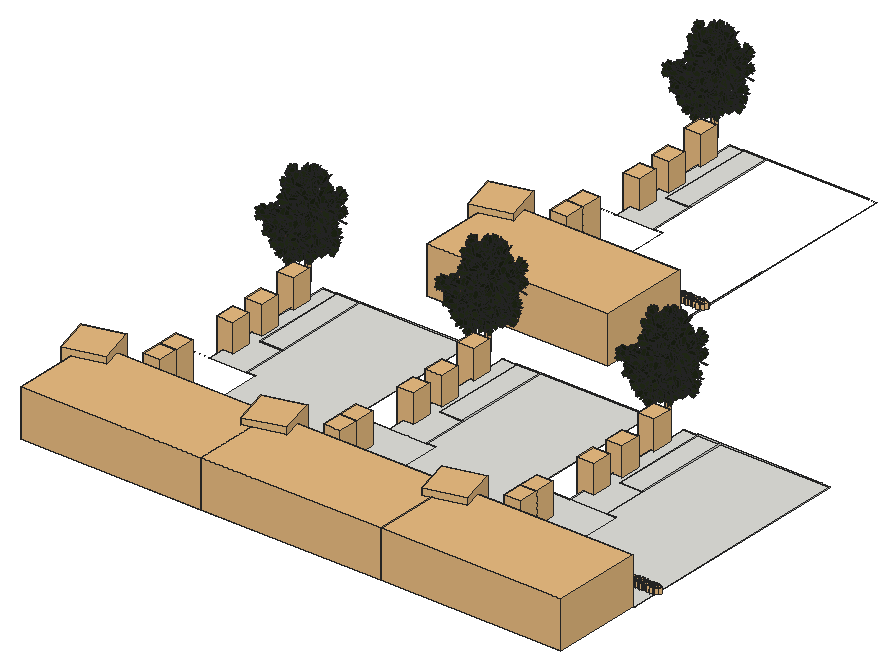
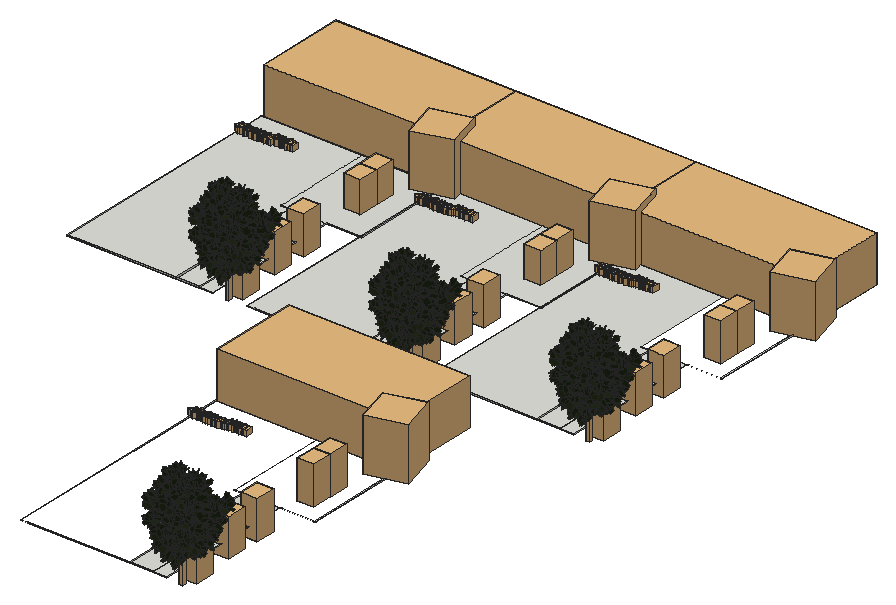
# SketchUp Ruby script. Lengths in inches.
U = 1.inch
M = Sketchup.active_model
def pt(a) = Geom::Point3d.new(a.map { |v| v * U })
def face(e, loops, mat)
  f = e.add_face(loops[0].map { |a| pt(a) })
  loops[1..].each { |l| e.add_face(l.map { |a| pt(a) }).erase! }
  f.material = f.back_material = mat if mat
  f
end
# faces: each face lists its corners as indices into pts; further lists are holes
def faces(e, pts, list, mat = nil) = list.each { |f| face(e, (f[0].is_a?(Array) ? f : [f]).map { |l| l.map { |i| pts[i] } }, mat) }
# xy, xz, yz: faces in a plane at the given z, y or x. An outline is a flat list of corners, or four numbers for a rectangle; further outlines are holes
def ring(l) = l.size == 4 ? [[l[0], l[1]], [l[2], l[1]], [l[2], l[3]], [l[0], l[3]]] : l.each_slice(2).to_a
def flat(e, list, mat, &to3) = list.each { |f| face(e, (f[0].is_a?(Array) ? f : [f]).map { |l| ring(l).map { |u, v| to3.(u, v) } }, mat) }
def xy(e, z, list, mat = nil) = flat(e, list, mat) { |x, y| [x, y, z] }
def xz(e, y, list, mat = nil) = flat(e, list, mat) { |x, z| [x, y, z] }
def yz(e, x, list, mat = nil) = flat(e, list, mat) { |y, z| [x, y, z] }
def lines(e, pts, list) = list.each { |a, b| e.add_line(pt(pts[a]), pt(pts[b])) }
# prism: a flat outline (further loops are holes) pulled along v
def prism(e, loops, v, mat = nil)
  f = face(e, loops, mat); d = Geom::Vector3d.new(v.map { |x| x * U })
  f.pushpull(f.normal.samedirection?(d) ? d.length : -d.length)
end
def box(e, o, s, mat = nil) = prism(e, [[o, [o[0] + s[0], o[1], o[2]], [o[0] + s[0], o[1] + s[1], o[2]], [o[0], o[1] + s[1], o[2]]]], [0, 0, s[2]], mat)
def at(x, y, z, deg = 0) = Geom::Transformation.translation(pt([x, y, z])) * Geom::Transformation.rotation(ORIGIN, Z_AXIS, deg.degrees)
def axes(o, x, y, z) = Geom::Transformation.new([*x, 0, *y, 0, *z, 0, *pt(o).to_a, 1])
def part(name) = M.definitions.add(name)
# library, detail: a bought-in or finely detailed component or shape, given as its bounding box
def library(name, o, s) = part(name).tap { |d| box(d.entities, o, s) }
def detail(e, o, s) = box(e.add_group.entities, o, s)
def put(e, d, t, mat = nil) = e.add_instance(d, t).tap { |i| i.material = mat if mat }
def group(e, t, mat = nil) = e.add_group.tap { |g| g.transformation = t; g.material = mat if mat }.entities
root = M.entities
M.materials.add("Green ash – green texture").color = [33, 41, 22]
M.materials.add("[Color_005]").color = [114, 114, 114]
M.materials.add("[Color_D09]").color = [86, 59, 49]
c1 = part("Component\#13")
xz(c1.entities,0,[[2.54,0,9.87,0.64,10.99,2.07,11.4,3.42,15.13,2.28,14.48,4.31,16.14,5.21,16.14,6.08,19.81,7.28,19.6,9.67,17.45,11.49,17.45,12.16,18.82,14.37,17.48,14.37,14.41,13.66,14.41,15.23,12.5625,17.49,9.84,15.21,8.9,13.85,7.74,13.625,7.35,12.68,6.87,13.02,6.35,12.27,5.92,10.47,4.2,7.42,2.84,6.89,0,2.38,0.07,1.59,2.8125,4.94,3.37,3.59,2.54,3.37,2.12,2.22]],"Green ash – green texture")
c2 = part("Component\#14")
xz(c2.entities,0,[[1.1,0,1.61,0,2.73,1.11,4.34,2.72,5.21,6.36,5.85,7.16,6.35,6.9375,6.85,8.05,8.03,8.05,8.625,9.25,10.11,11.7,9.56,13.83,9.56,15.84,7.83,15.84,6.03,14.37,5.31,16.54,4.4375,17.39,1.45,14.31,0,9.15,1.4,5.18,3.01,6.08,1.98,1.39]],"Green ash – green texture")
c3 = part("Component\#16")
put(c3.entities,c1,axes([0,7.77,0],[1,0,0],[0,0.89571,0.44464],[0,-0.44464,0.89571]))
put(c3.entities,c2,axes([2.15,6.37,5.26],[0.57629,-0.80824,0.12095],[0.79263,0.51673,-0.3236],[0.19905,0.28236,0.93843]))
c4 = part("Component\#4")
put(c4.entities,c3,axes([-4.97,-3.22,4.05],[0.69883,-0.69034,0.18725],[0.53248,0.3273,-0.7806],[0.47759,0.64522,0.59632]))
c5 = part("Component\#5")
put(c5.entities,c4,axes([0,5.2,2.2],[1,0,0],[0,0.90259,0.43051],[0,-0.43051,0.90259]))
c6 = part("leaf group 2")
put(c6.entities,c5,axes([-11.99,4.41,-4.35],[2.22014,-0.82385,1.14017],[1.36501,1.77637,-1.37441],[-0.33979,1.75315,1.92841]))
c7 = part("Component\#6")
put(c7.entities,c6,axes([-5.27,11.65,1.68],[-0.48323,0.10636,-0.43072],[-0.11515,-0.64511,-0.03012],[-0.42845,0.05342,0.49388]))
c8 = part("Component\#15")
xz(c8.entities,0,[[0.64,0,0,0.1875,4.21,2.81,8.59,4.11,12.8,4.11,19.57,2.81,12.8,3.73,8.59,3.73,4.21,2.3125]],"[Color_D09]")
c9 = part("Leaf cluster")
put(c9.entities,c7,axes([23.53,12.57,24.85],[0.06536,-0.90475,-0.42089],[0.61791,-0.2945,0.72901],[-0.78353,-0.30772,0.53981]))
put(c9.entities,c7,axes([22.7,12.25,24.83],[-0.47146,-0.89493,0.11311],[0.80135,-0.48549,-0.35888],[0.36776,-0.0521,0.90651]))
put(c9.entities,c7,axes([24.25,0.65,20.83],[0.8253,-0.50372,0.24924],[0.23848,0.71461,0.65749],[-0.51157,-0.48438,0.71194]))
put(c9.entities,c7,axes([23.54,-2.45,18.63],[0.04689,-0.92492,0.3511],[0.72122,-0.28285,-0.64421],[0.71641,0.2674,0.65188]))
put(c9.entities,c7,axes([22.39,16.15,27.04],[-0.5311,-0.82173,0.2419],[0.41574,0.01583,0.89559],[-0.77461,0.50499,0.40813]))
put(c9.entities,c8,axes([22.76,-5.09,13.48],[0,1.66539,0.44624],[-1.72414,0,0],[0,-0.44624,1.66539]))
c10 = part("Component\#12")
p = [[0,0,0.13],[0.41,0.77,0],[4.07,2.79,10.125],[3.73,2.15,10.23],[7.66,4.77,23.875],[7.4,4.27,23.96],
  [8.6875,5.26,35.99],[8.5,4.91,36.05],[8.32,4.9375,46.95],[8.21,4.74,46.98]]
faces(c10.entities,p,[[0,1,2,3],[3,2,4,5],[4,6,7,5],[6,8,9,7]],"[Color_005]")
c11 = part("Component\#8")
put(c11.entities,c10,axes([3.13,0.17,-0.45],[3.38032,6.88592,0.52481],[-5.85488,3.97559,0.303],[0,-1.35912,3.54524]))
put(c11.entities,c7,axes([0.37,31.375,148.94],[0.47772,0.64064,-1.51139],[2.85768,-0.62659,0.20284],[-0.43926,-3.3797,-0.3241]))
c12 = part("Leafy branch")
put(c12.entities,c9,axes([28.11,72.66,46.26],[0.77413,-0.41274,-0.47998],[0.6311,0.56229,0.53435],[0.04934,-0.71657,0.69577]))
put(c12.entities,c9,axes([31.25,3.94,9.17],[0.73236,0.67893,0.05208],[-0.46223,0.55185,-0.69413],[-0.5,0.48428,0.71797]))
put(c12.entities,c9,axes([20.16,84.84,57.95],[0.96628,0.19619,0.16678],[-0.2575,0.73909,0.62245],[-0.00115,-0.6444,0.76469]))
put(c12.entities,c9,axes([30.13,29.18,11.93],[0.86603,0.2796,0.41452],[0,0.82904,-0.55919],[-0.5,0.48428,0.71797]))
put(c12.entities,c9,axes([47.67,28.63,-3.7],[0.1205,-0.71255,0.69119],[0.96646,0.24327,0.08231],[-0.2268,0.65809,0.71797]))
put(c12.entities,c9,axes([48.76,50.64,76.31],[-0.6716,0.46861,-0.57389],[0.01402,0.78248,0.62252],[0.74078,0.41004,-0.53209]))
put(c12.entities,c11,axes([42.34,0,10.34],[0.39368,0,0],[0,0.22544,-0.24092],[0,0.54032,0.50562]))
put(c12.entities,c9,axes([64.51,80.82,101.08],[-0.99604,0.06562,-0.06004],[-0.0106,0.58266,0.81265],[0.08831,0.81006,-0.57966]))
c13 = library("Component\#9",[-6.35,9.4375,-76.57],[12.56,13.68,315.77])
c14 = part("Component\#11")
put(c14.entities,c9,axes([-3.64,36.17,23.18],[0.95801,0.10249,0.26779],[-0.28581,0.41631,0.86313],[-0.02302,-0.90343,0.42812]))
put(c14.entities,c9,axes([13.16,55.79,39.92],[0.70711,-0.61725,0.34497],[0,0.48786,0.87292],[-0.70711,-0.61725,0.34497]))
put(c14.entities,c11,axes([18.8125,5.17,0.46],[0.25503,0,0],[0,0.20007,-0.0752],[0,0.16866,0.44872]))
put(c14.entities,c9,axes([23.62,-10.17,21.5],[-0.56253,0.81775,0.12181],[0.38738,0.13053,0.91263],[0.73041,0.56057,-0.39021]))
put(c14.entities,c9,axes([45.18,27.18,68.96],[-0.96593,-0.22593,0.12627],[0.12295,0.02876,0.992],[-0.22775,0.97372,0]))
c15 = part("Component\#10")
put(c15.entities,c11,axes([21.47,3.93,0.22],[0.25503,0,0],[0,0.21068,-0.03601],[0,0.08077,0.47252]))
put(c15.entities,c9,axes([-4.05,13.6875,55.34],[0.70711,0.70373,-0.069],[0,0.09758,0.99523],[0.70711,-0.70373,0.069]))
put(c15.entities,c9,axes([6.52,33.54,18.07],[0.92587,-0.37604,0.03687],[0,0.09758,0.99523],[-0.37784,-0.92145,0.09035]))
c16 = part("Component\#18")
put(c16.entities,c9,axes([26.17,74.02,40.56],[0.25882,-0.64004,0.72344],[0,0.74896,0.66262],[-0.96593,-0.1715,0.19384]))
put(c16.entities,c9,axes([6.38,24.03,55.81],[-0.04786,0.8645,-0.50035],[0.15558,0.50126,0.85119],[0.98666,-0.03711,-0.15849]))
put(c16.entities,c11,axes([17.68,0,1.01],[0.32282,0,0],[0,0.21407,-0.16545],[0,0.37107,0.48011]))
put(c16.entities,c9,axes([-9.1875,31.15,28.07],[0.82314,0.37626,-0.42529],[0,0.74896,0.66262],[0.56784,-0.54543,0.61649]))
put(c16.entities,c9,axes([0.54,-12.07,9.94],[0.19622,0.90478,-0.37799],[-0.67396,0.40444,0.61823],[0.71224,0.13344,0.68914]))
put(c16.entities,c9,axes([7.34,9.15,39.57],[0.05153,0.73872,-0.67204],[0.38679,0.60565,0.6954],[0.92072,-0.29578,-0.25452]))
put(c16.entities,c9,axes([36.2,51.23,15.73],[-0.18626,-0.35374,0.91661],[-0.31641,0.90483,0.2849],[-0.93016,-0.23696,-0.28046]))
c17 = part("Tree")
put(c17.entities,c12,axes([-22.29,52.36,216.76],[0.38964,-1.07313,-0.10036],[1.06809,0.37236,0.19631],[-0.13881,-0.14712,1.22884]))
put(c17.entities,c12,axes([59.83,6.78,230.57],[-1.28826,-0.23008,-0.3647],[0.05148,-1.22938,0.51215],[-0.34663,0.55136,1.25774]))
put(c17.entities,c13,axes([-2.16,-18.04,104.22],[1.30157,0,0],[0,1.30157,0],[0,0,1.36111]))
put(c17.entities,c12,axes([-55.8,4.2,115.32],[1.30157,0,0],[0,1.29536,0.19359],[0,-0.26855,1.38538]))
put(c17.entities,c12,axes([5.36,-52.22,156.04],[-0.23532,1.19719,-0.71362],[-1.32974,0,0.39335],[0.40758,0.6912,1.23603]))
put(c17.entities,c14,axes([-20.09,22.57,317.7],[0,-1.33697,0],[1.33697,0,0],[0,0,1.4573]))
put(c17.entities,c12,axes([44.2,-31.84,172.82],[-1.11894,0.85085,0],[-0.85085,-1.11894,0],[0,0,1.53221]))
put(c17.entities,c12,axes([-10.2,63.7,119.93],[0.28716,-1.46366,0],[1.41378,0.27737,0.38604],[-0.41292,-0.08101,1.5704]))
put(c17.entities,c12,axes([-29.03,-40.72,232.79],[0.5211,0.98898,-0.38718],[-1.02974,0.58664,0.11255],[0.35577,0.28216,1.19957]))
put(c17.entities,c12,axes([44.92,21.7,135.38],[-1.05627,-0.44294,0],[0.44294,-1.05627,0],[0,0,1.24847]))
put(c17.entities,c14,axes([-32.94,-0.59,304.82],[1.2814,-0.22825,0],[0.22825,1.2814,0],[0,0,1.41871]))
put(c17.entities,c14,axes([0.6,-31.29,315.98],[0.13082,1.33422,0],[-1.33422,0.13082,0],[0,0,1.46127]))
put(c17.entities,c14,axes([21.3,1.66,315.16],[-1.25722,0.32198,-0.09905],[-0.32539,-1.26867,0.00612],[-0.08719,0.09194,1.40547]))
put(c17.entities,c15,axes([-19,30.84,372.72],[0.65078,-1.12719,0],[1.12719,0.65078,0],[0,0,1.41871]))
put(c17.entities,c15,axes([14.39,-16.125,357],[-0.73695,1.06095,0.15933],[-1.03698,-0.75397,0.2242],[0.29981,0,1.38667]))
put(c17.entities,c16,axes([-5.9,-20.03,270.39],[0,1.47598,0],[-1.4157,0,0.41751],[0.45509,0,1.54311]))
put(c17.entities,c16,axes([-18.4375,22.18,263.88],[0.84243,-1.42226,-0.32685],[1.40385,0.7063,0.64743],[-0.37678,-0.54841,1.68147]))
put(c17.entities,c16,axes([-29.32,4.9,283.41],[1.35363,0,0],[0,1.33841,0.20242],[0,-0.22063,1.45887]))
put(c17.entities,c16,axes([17.31,11.65,257.52],[-1.14969,-0.5642,-0.25322],[0.46017,-1.12719,0.50159],[-0.40066,0.32434,1.3027]))
put(c17.entities,c16,axes([16.3,15.3125,240.45],[-0.98541,-0.85203,0.68095],[1.00747,-1.01506,0.22317],[0.31818,0.5753,1.40228]))
put(c17.entities,c12,axes([-46.75,22.93,206.12],[1.08363,-0.37101,0],[0.37101,1.08363,0],[0,0,1.24847]))
put(c17.entities,c12,axes([41.1,-35.18,99.125],[-1.05556,0.85173,0.25344],[-0.84493,-1.04965,0.12953],[0.39153,-0.09409,1.38106]))
c18 = library("Potted plant",[-29.7,0,-10.87],[31.67,38.52,72.45])
c19 = library("Obj_000004",[-25.54,-25.36,-14.31],[50.67,50.64,41.42])
c20 = library("Palm tree",[-4.09,-4.52,0],[193.52,193.51,258.93])
c21 = part("Palm+Tree")
put(c21.entities,c20,at(25.51,-21.81,0,15))
c22 = library("BPJ-Road5D",[0,0,1],[442,720,229.125])
xy(root,-25.5625,[[68.91,0,75.99,505.3125],[468.02,0,468.02,505.3125,424.39,505.3125,424.39,1201.875,962.46,1201.875,962.46,505.3125,955.37,505.3125,955.37,0],[955.37,0,962.46,505.3125],[962.46,0,1354.48,505.3125],[1354.48,0,1354.48,505.3125,1310.86,505.3125,1310.86,1201.875,1848.92,1201.875,1848.92,505.3125,1841.83,505.3125,1841.83,0],
  [1841.83,0,1848.92,505.3125],[1848.92,0,2240.94,505.3125],[2240.94,0,2240.94,505.3125,2197.32,505.3125,2197.32,1201.875,2735.38,1201.875,2735.38,0],[241.33,505.3125,241.33,1201.875,310.02,1201.875,310.02,726.125,424.39,726.125,424.39,505.3125],[1127.79,505.3125,1127.79,1201.875,1196.48,1201.875,1196.48,726.125,1310.86,726.125,1310.86,505.3125],
  [2014.26,505.3125,2014.26,1201.875,2082.95,1201.875,2082.95,726.125,2197.32,726.125,2197.32,505.3125],[310.02,726.125,424.39,1201.875],[1196.48,726.125,1310.86,1201.875],[2082.95,726.125,2197.32,1201.875],[587.64,1851.99,594.72,2357.31],
  [1474.1,1851.99,1481.1875,2357.31],[760.06,2357.31,760.06,3053.87,828.75,3053.87,828.75,2578.12,943.125,2578.12,943.125,2357.31],[828.75,2578.12,943.125,3053.87]])
xz(root,0,[[75.99,-25.5625,955.37,-23.875],[955.37,-25.5625,962.46,-23.875],[962.46,-25.5625,1841.83,-23.875],[1841.83,-25.5625,1848.92,-23.875],[1848.92,-25.5625,2735.38,-23.875]])
xz(root,505.3125,[[68.91,-25.5625,241.33,-23.875],[424.39,-25.5625,468.02,-23.875],[955.37,-25.5625,1127.79,-23.875],[1310.86,-25.5625,1354.48,-23.875],[1841.83,-25.5625,2014.26,-23.875],
  [2197.32,-25.5625,2240.94,-23.875]])
xz(root,726.125,[[310.02,-25.5625,424.39,-23.875],[1196.48,-25.5625,1310.86,-23.875],[2082.95,-25.5625,2197.32,-23.875]])
xz(root,1201.875,[[241.33,-25.5625,310.02,-23.875],[310.02,-25.5625,424.39,-19.75],[424.39,-25.5625,916.77,-19.75],[916.77,-25.5625,916.77,-19.75,923.77,-19.75,923.77,-23.875,962.46,-23.875,962.46,-25.5625],[1127.79,-25.5625,1196.48,-23.875],
  [1196.48,-25.5625,1310.86,-19.75],[1310.86,-25.5625,1803.23,-19.75],[1803.23,-25.5625,1803.23,-19.75,1810.23,-19.75,1810.23,-23.875,1848.92,-23.875,1848.92,-25.5625],[2014.26,-25.5625,2082.95,-23.875],[2082.95,-25.5625,2197.32,-19.75],
  [2197.32,-25.5625,2689.7,-19.75],[2689.7,-25.5625,2689.7,-19.75,2696.7,-19.75,2696.7,-23.875,2735.38,-23.875,2735.38,-25.5625]])
xz(root,1851.99,[[1474.1,-25.5625,1481.1875,-23.875]])
xz(root,2357.31,[[587.64,-25.5625,760.06,-23.875],[943.125,-25.5625,986.75,-23.875]])
xz(root,2578.12,[[828.75,-25.5625,943.125,-23.875]])
xz(root,3053.87,[[760.06,-25.5625,828.75,-23.875],[828.75,-25.5625,943.125,-19.75],[943.125,-25.5625,1435.5,-19.75],[1435.5,-25.5625,1435.5,-19.75,1442.5,-19.75,1442.5,-23.875,1481.1875,-23.875,1481.1875,-25.5625]])
yz(root,68.91,[[0,-25.5625,0,-23.875,143.39,-23.875,143.39,-19.75,164.82,-19.75,164.82,-23.875,505.3125,-23.875,505.3125,-25.5625]])
yz(root,241.33,[[505.3125,-25.5625,1201.875,-23.875]])
yz(root,310.02,[[726.125,-25.5625,1201.875,-23.875]])
yz(root,424.39,[[505.3125,-25.5625,726.125,-23.875],[726.125,-25.5625,1201.875,-19.75]])
yz(root,587.64,[[1851.99,-25.5625,1851.99,-23.875,1995.38,-23.875,1995.38,-19.75,2016.82,-19.75,2016.82,-23.875,2357.31,-23.875,2357.31,-25.5625]])
yz(root,760.06,[[2357.31,-25.5625,3053.87,-23.875]])
yz(root,828.75,[[2578.12,-25.5625,3053.87,-23.875]])
yz(root,943.125,[[2357.31,-25.5625,2578.12,-23.875],[2578.12,-25.5625,3053.87,-19.75]])
yz(root,955.37,[[0,-25.5625,0,-23.875,143.39,-23.875,143.39,-19.75,164.82,-19.75,164.82,-23.875,505.3125,-23.875,505.3125,-25.5625]])
yz(root,962.46,[[0,-25.5625,1201.875,-23.875]])
yz(root,1127.79,[[505.3125,-25.5625,1201.875,-23.875]])
yz(root,1196.48,[[726.125,-25.5625,1201.875,-23.875]])
yz(root,1310.86,[[505.3125,-25.5625,726.125,-23.875],[726.125,-25.5625,1201.875,-19.75]])
yz(root,1481.1875,[[1851.99,-25.5625,3053.87,-23.875]])
yz(root,1841.83,[[0,-25.5625,0,-23.875,143.39,-23.875,143.39,-19.75,164.82,-19.75,164.82,-23.875,505.3125,-23.875,505.3125,-25.5625]])
yz(root,1848.92,[[0,-25.5625,1201.875,-23.875]])
yz(root,2014.26,[[505.3125,-25.5625,1201.875,-23.875]])
yz(root,2082.95,[[726.125,-25.5625,1201.875,-23.875]])
yz(root,2197.32,[[505.3125,-25.5625,726.125,-23.875],[726.125,-25.5625,1201.875,-19.75]])
yz(root,2735.38,[[0,-25.5625,1201.875,-23.875]])
p = [[986.75,1851.99,-25.5625],[594.72,1851.99,-25.5625],[986.75,2357.31,-25.5625],[1474.1,1851.99,-25.5625],[594.72,1851.99,-23.875]]
lines(root,p,[[0,1],[2,0],[0,3],[4,1]])
put(root,c17,at(1052.17,1201.875,-23.875))
put(root,c17,at(1938.63,1201.875,-23.875))
put(root,c17,at(165.7,1201.875,-23.875))
put(root,c17,at(684.43,3053.87,-23.875))
put(root,c18,axes([1169.43,591.59,-49.33],[2.592,0,0],[0,2.592,0],[0,0,2.592]))
put(root,c18,axes([1169.43,767.71,-49.33],[2.592,0,0],[0,2.592,0],[0,0,2.592]))
put(root,c18,axes([2055.89,767.71,-49.33],[2.592,0,0],[0,2.592,0],[0,0,2.592]))
put(root,c18,axes([2055.89,591.59,-49.33],[2.592,0,0],[0,2.592,0],[0,0,2.592]))
put(root,c18,axes([282.96,767.71,-49.33],[2.592,0,0],[0,2.592,0],[0,0,2.592]))
put(root,c18,axes([282.96,591.59,-49.33],[2.592,0,0],[0,2.592,0],[0,0,2.592]))
put(root,c18,axes([801.69,2619.71,-49.33],[2.592,0,0],[0,2.592,0],[0,0,2.592]))
put(root,c18,axes([801.69,2443.58,-49.33],[2.592,0,0],[0,2.592,0],[0,0,2.592]))
put(root,c18,axes([1137.61,1003.39,-45.74],[2.592,0,0],[0,2.592,0],[0,0,2.592]))
put(root,c18,axes([2024.08,1003.39,-45.74],[2.592,0,0],[0,2.592,0],[0,0,2.592]))
put(root,c18,axes([251.15,1003.39,-45.74],[2.592,0,0],[0,2.592,0],[0,0,2.592]))
put(root,c18,axes([769.88,2855.38,-45.74],[2.592,0,0],[0,2.592,0],[0,0,2.592]))
put(root,c18,axes([1150.69,266.71,-33.56],[2.592,0,0],[0,2.592,0],[0,0,2.592]))
put(root,c18,axes([1150.69,164.82,-33.56],[2.592,0,0],[0,2.592,0],[0,0,2.592]))
put(root,c18,axes([782.96,2016.82,-33.56],[2.592,0,0],[0,2.592,0],[0,0,2.592]))
put(root,c18,axes([782.96,2118.7,-33.56],[2.592,0,0],[0,2.592,0],[0,0,2.592]))
put(root,c18,axes([2037.16,266.71,-33.56],[2.592,0,0],[0,2.592,0],[0,0,2.592]))
put(root,c18,axes([264.23,266.71,-33.56],[2.592,0,0],[0,2.592,0],[0,0,2.592]))
put(root,c18,axes([2037.16,164.82,-33.56],[2.592,0,0],[0,2.592,0],[0,0,2.592]))
put(root,c18,axes([264.23,164.82,-33.56],[2.592,0,0],[0,2.592,0],[0,0,2.592]))
put(root,c19,axes([1646.38,130.18,-17.02],[0.45255,0.45255,-0.00035],[-0.45255,0.45255,0.00015],[0.00035,0.00015,0.64]))
put(root,c19,axes([1630.48,130.4,-17.02],[-0.16941,0.61717,-0.00035],[-0.61717,-0.16941,0.00015],[0.00005,0.00038,0.64]))
put(root,c19,axes([1614.64,130.18,-17.02],[0.45255,0.45255,-0.00035],[-0.45255,0.45255,0.00015],[0.00035,0.00015,0.64]))
put(root,c19,axes([1676.95,129.48,-17.02],[0.34155,0.54124,-0.00035],[-0.54124,0.34155,0.00015],[0.00031,0.00022,0.64]))
put(root,c19,axes([1662.26,130.18,-17.02],[0.45255,0.45255,-0.00035],[-0.45255,0.45255,0.00015],[0.00035,0.00015,0.64]))
put(root,c19,axes([2548.72,130.18,-17.02],[0.45255,0.45255,-0.00035],[-0.45255,0.45255,0.00015],[0.00035,0.00015,0.64]))
put(root,c19,axes([2563.41,129.48,-17.02],[0.34155,0.54124,-0.00035],[-0.54124,0.34155,0.00015],[0.00031,0.00022,0.64]))
put(root,c19,axes([2501.1,130.18,-17.02],[0.45255,0.45255,-0.00035],[-0.45255,0.45255,0.00015],[0.00035,0.00015,0.64]))
put(root,c19,axes([2532.85,130.18,-17.02],[0.45255,0.45255,-0.00035],[-0.45255,0.45255,0.00015],[0.00035,0.00015,0.64]))
put(root,c19,axes([2516.95,130.4,-17.02],[-0.16941,0.61717,-0.00035],[-0.61717,-0.16941,0.00015],[0.00005,0.00038,0.64]))
put(root,c19,axes([790.48,129.48,-17.02],[0.34155,0.54124,-0.00035],[-0.54124,0.34155,0.00015],[0.00031,0.00022,0.64]))
put(root,c19,axes([759.92,130.18,-17.02],[0.45255,0.45255,-0.00035],[-0.45255,0.45255,0.00015],[0.00035,0.00015,0.64]))
put(root,c19,axes([775.79,130.18,-17.02],[0.45255,0.45255,-0.00035],[-0.45255,0.45255,0.00015],[0.00035,0.00015,0.64]))
put(root,c19,axes([728.17,130.18,-17.02],[0.45255,0.45255,-0.00035],[-0.45255,0.45255,0.00015],[0.00035,0.00015,0.64]))
put(root,c19,axes([744.02,130.4,-17.02],[-0.16941,0.61717,-0.00035],[-0.61717,-0.16941,0.00015],[0.00005,0.00038,0.64]))
put(root,c19,axes([1294.53,1982.18,-17.02],[0.45255,0.45255,-0.00035],[-0.45255,0.45255,0.00015],[0.00035,0.00015,0.64]))
put(root,c19,axes([1246.9,1982.18,-17.02],[0.45255,0.45255,-0.00035],[-0.45255,0.45255,0.00015],[0.00035,0.00015,0.64]))
put(root,c19,axes([1262.75,1982.39,-17.02],[-0.16941,0.61717,-0.00035],[-0.61717,-0.16941,0.00015],[0.00005,0.00038,0.64]))
put(root,c19,axes([1309.22,1981.47,-17.02],[0.34155,0.54124,-0.00035],[-0.54124,0.34155,0.00015],[0.00031,0.00022,0.64]))
put(root,c19,axes([1278.65,1982.18,-17.02],[0.45255,0.45255,-0.00035],[-0.45255,0.45255,0.00015],[0.00035,0.00015,0.64]))
put(root,c19,axes([1677.44,130.52,-17.02],[0.28256,0.57425,0],[-0.57425,0.28256,0],[0,0,0.64]))
put(root,c19,axes([1598.35,130.26,-17.02],[0.64,0,0],[0,0.64,0],[0,0,0.64]))
put(root,c19,axes([1614.23,130.26,-17.02],[0.64,0,0],[0,0.64,0],[0,0,0.64]))
put(root,c19,axes([1645.97,130.26,-17.02],[0.64,0,0],[0,0.64,0],[0,0,0.64]))
put(root,c19,axes([1630.48,130.71,-17.02],[-0.15049,0.62206,0],[-0.62206,-0.15049,0],[0,0,0.64]))
put(root,c19,axes([1661.85,130.26,-17.02],[0.64,0,0],[0,0.64,0],[0,0,0.64]))
put(root,c19,axes([2516.95,130.71,-17.02],[-0.15049,0.62206,0],[-0.62206,-0.15049,0],[0,0,0.64]))
put(root,c19,axes([2548.3125,130.26,-17.02],[0.64,0,0],[0,0.64,0],[0,0,0.64]))
put(root,c19,axes([2532.4375,130.26,-17.02],[0.64,0,0],[0,0.64,0],[0,0,0.64]))
put(root,c19,axes([2563.9,130.52,-17.02],[0.28256,0.57425,0],[-0.57425,0.28256,0],[0,0,0.64]))
put(root,c19,axes([2484.82,130.26,-17.02],[0.64,0,0],[0,0.64,0],[0,0,0.64]))
put(root,c19,axes([2500.69,130.26,-17.02],[0.64,0,0],[0,0.64,0],[0,0,0.64]))
put(root,c19,axes([790.97,130.52,-17.02],[0.28256,0.57425,0],[-0.57425,0.28256,0],[0,0,0.64]))
put(root,c19,axes([711.89,130.26,-17.02],[0.64,0,0],[0,0.64,0],[0,0,0.64]))
put(root,c19,axes([727.76,130.26,-17.02],[0.64,0,0],[0,0.64,0],[0,0,0.64]))
put(root,c19,axes([759.51,130.26,-17.02],[0.64,0,0],[0,0.64,0],[0,0,0.64]))
put(root,c19,axes([744.02,130.71,-17.02],[-0.15049,0.62206,0],[-0.62206,-0.15049,0],[0,0,0.64]))
put(root,c19,axes([775.38,130.26,-17.02],[0.64,0,0],[0,0.64,0],[0,0,0.64]))
put(root,c19,axes([1294.12,1982.25,-17.02],[0.64,0,0],[0,0.64,0],[0,0,0.64]))
put(root,c19,axes([1262.75,1982.71,-17.02],[-0.15049,0.62206,0],[-0.62206,-0.15049,0],[0,0,0.64]))
put(root,c19,axes([1246.49,1982.25,-17.02],[0.64,0,0],[0,0.64,0],[0,0,0.64]))
put(root,c19,axes([1278.24,1982.25,-17.02],[0.64,0,0],[0,0.64,0],[0,0,0.64]))
put(root,c19,axes([1309.7,1982.52,-17.02],[0.28256,0.57425,0],[-0.57425,0.28256,0],[0,0,0.64]))
put(root,c19,axes([1230.62,1982.25,-17.02],[0.64,0,0],[0,0.64,0],[0,0,0.64]))
put(root,c21,at(890.73,-113.71,-26.05))
put(root,c21,at(522.99,1738.29,-26.05))
put(root,c21,at(1777.19,-113.71,-26.05))
put(root,c21,at(4.26,-113.71,-26.05))
put(root,c22,axes([1841.83,-442,-26.5625],[0,1,0],[-1.2312,0,0],[0,0,1]))
put(root,c22,axes([2728.3,-442,-26.5625],[0,1,0],[-1.2312,0,0],[0,0,1]))
put(root,c22,axes([955.37,-442,-26.5625],[0,1,0],[-1.2312,0,0],[0,0,1]))
put(root,c22,axes([1474.1,1409.99,-26.5625],[0,1,0],[-1.2312,0,0],[0,0,1]))
put(root,c19,axes([1756.1,144.13,-16.22],[0.45255,0.45255,-0.00035],[-0.45255,0.45255,0.00015],[0.00035,0.00015,0.64]))
put(root,c19,axes([1770.79,143.43,-16.22],[0.34155,0.54124,-0.00035],[-0.54124,0.34155,0.00015],[0.00031,0.00022,0.64]))
put(root,c19,axes([1708.47,144.13,-16.22],[0.45255,0.45255,-0.00035],[-0.45255,0.45255,0.00015],[0.00035,0.00015,0.64]))
put(root,c19,axes([1740.22,144.13,-16.22],[0.45255,0.45255,-0.00035],[-0.45255,0.45255,0.00015],[0.00035,0.00015,0.64]))
put(root,c19,axes([1724.32,144.35,-16.22],[-0.16941,0.61717,-0.00035],[-0.61717,-0.16941,0.00015],[0.00005,0.00038,0.64]))
put(root,c19,axes([1826.47,144.13,-16.22],[0.45255,0.45255,-0.00035],[-0.45255,0.45255,0.00015],[0.00035,0.00015,0.64]))
put(root,c19,axes([1841.16,143.43,-16.22],[0.34155,0.54124,-0.00035],[-0.54124,0.34155,0.00015],[0.00031,0.00022,0.64]))
put(root,c19,axes([1778.85,144.13,-16.22],[0.45255,0.45255,-0.00035],[-0.45255,0.45255,0.00015],[0.00035,0.00015,0.64]))
put(root,c19,axes([1810.6,144.13,-16.22],[0.45255,0.45255,-0.00035],[-0.45255,0.45255,0.00015],[0.00035,0.00015,0.64]))
put(root,c19,axes([1794.7,144.35,-16.22],[-0.16941,0.61717,-0.00035],[-0.61717,-0.16941,0.00015],[0.00005,0.00038,0.64]))
put(root,c19,axes([2697.06,144.13,-16.22],[0.45255,0.45255,-0.00035],[-0.45255,0.45255,0.00015],[0.00035,0.00015,0.64]))
put(root,c19,axes([2665.3125,144.13,-16.22],[0.45255,0.45255,-0.00035],[-0.45255,0.45255,0.00015],[0.00035,0.00015,0.64]))
put(root,c19,axes([2681.16,144.35,-16.22],[-0.16941,0.61717,-0.00035],[-0.61717,-0.16941,0.00015],[0.00005,0.00038,0.64]))
put(root,c19,axes([2712.93,144.13,-16.22],[0.45255,0.45255,-0.00035],[-0.45255,0.45255,0.00015],[0.00035,0.00015,0.64]))
put(root,c19,axes([2727.625,143.43,-16.22],[0.34155,0.54124,-0.00035],[-0.54124,0.34155,0.00015],[0.00031,0.00022,0.64]))
put(root,c19,axes([2642.56,144.13,-16.22],[0.45255,0.45255,-0.00035],[-0.45255,0.45255,0.00015],[0.00035,0.00015,0.64]))
put(root,c19,axes([2657.25,143.43,-16.22],[0.34155,0.54124,-0.00035],[-0.54124,0.34155,0.00015],[0.00031,0.00022,0.64]))
put(root,c19,axes([2594.9375,144.13,-16.22],[0.45255,0.45255,-0.00035],[-0.45255,0.45255,0.00015],[0.00035,0.00015,0.64]))
put(root,c19,axes([2626.69,144.13,-16.22],[0.45255,0.45255,-0.00035],[-0.45255,0.45255,0.00015],[0.00035,0.00015,0.64]))
put(root,c19,axes([2610.79,144.35,-16.22],[-0.16941,0.61717,-0.00035],[-0.61717,-0.16941,0.00015],[0.00005,0.00038,0.64]))
put(root,c19,axes([892.38,144.13,-16.22],[0.45255,0.45255,-0.00035],[-0.45255,0.45255,0.00015],[0.00035,0.00015,0.64]))
put(root,c19,axes([924.13,144.13,-16.22],[0.45255,0.45255,-0.00035],[-0.45255,0.45255,0.00015],[0.00035,0.00015,0.64]))
put(root,c19,axes([908.23,144.35,-16.22],[-0.16941,0.61717,-0.00035],[-0.61717,-0.16941,0.00015],[0.00005,0.00038,0.64]))
put(root,c19,axes([940.01,144.13,-16.22],[0.45255,0.45255,-0.00035],[-0.45255,0.45255,0.00015],[0.00035,0.00015,0.64]))
put(root,c19,axes([954.7,143.43,-16.22],[0.34155,0.54124,-0.00035],[-0.54124,0.34155,0.00015],[0.00031,0.00022,0.64]))
put(root,c19,axes([822.01,144.13,-16.22],[0.45255,0.45255,-0.00035],[-0.45255,0.45255,0.00015],[0.00035,0.00015,0.64]))
put(root,c19,axes([837.86,144.35,-16.22],[-0.16941,0.61717,-0.00035],[-0.61717,-0.16941,0.00015],[0.00005,0.00038,0.64]))
put(root,c19,axes([869.63,144.13,-16.22],[0.45255,0.45255,-0.00035],[-0.45255,0.45255,0.00015],[0.00035,0.00015,0.64]))
put(root,c19,axes([884.32,143.43,-16.22],[0.34155,0.54124,-0.00035],[-0.54124,0.34155,0.00015],[0.00031,0.00022,0.64]))
put(root,c19,axes([853.76,144.13,-16.22],[0.45255,0.45255,-0.00035],[-0.45255,0.45255,0.00015],[0.00035,0.00015,0.64]))
put(root,c19,axes([1442.86,1996.125,-16.22],[0.45255,0.45255,-0.00035],[-0.45255,0.45255,0.00015],[0.00035,0.00015,0.64]))
put(root,c19,axes([1340.74,1996.125,-16.22],[0.45255,0.45255,-0.00035],[-0.45255,0.45255,0.00015],[0.00035,0.00015,0.64]))
put(root,c19,axes([1411.12,1996.125,-16.22],[0.45255,0.45255,-0.00035],[-0.45255,0.45255,0.00015],[0.00035,0.00015,0.64]))
put(root,c19,axes([1458.74,1996.125,-16.22],[0.45255,0.45255,-0.00035],[-0.45255,0.45255,0.00015],[0.00035,0.00015,0.64]))
put(root,c19,axes([1473.43,1995.42,-16.22],[0.34155,0.54124,-0.00035],[-0.54124,0.34155,0.00015],[0.00031,0.00022,0.64]))
put(root,c19,axes([1388.36,1996.125,-16.22],[0.45255,0.45255,-0.00035],[-0.45255,0.45255,0.00015],[0.00035,0.00015,0.64]))
put(root,c19,axes([1356.59,1996.34,-16.22],[-0.16941,0.61717,-0.00035],[-0.61717,-0.16941,0.00015],[0.00005,0.00038,0.64]))
put(root,c19,axes([1403.05,1995.42,-16.22],[0.34155,0.54124,-0.00035],[-0.54124,0.34155,0.00015],[0.00031,0.00022,0.64]))
put(root,c19,axes([1426.96,1996.34,-16.22],[-0.16941,0.61717,-0.00035],[-0.61717,-0.16941,0.00015],[0.00005,0.00038,0.64]))
put(root,c19,axes([1372.49,1996.125,-16.22],[0.45255,0.45255,-0.00035],[-0.45255,0.45255,0.00015],[0.00035,0.00015,0.64]))
put(root,c19,axes([1724.32,144.66,-16.22],[-0.15049,0.62206,0],[-0.62206,-0.15049,0],[0,0,0.64]))
put(root,c19,axes([1755.6875,144.21,-16.22],[0.64,0,0],[0,0.64,0],[0,0,0.64]))
put(root,c19,axes([1739.8125,144.21,-16.22],[0.64,0,0],[0,0.64,0],[0,0,0.64]))
put(root,c19,axes([1771.27,144.47,-16.22],[0.28256,0.57425,0],[-0.57425,0.28256,0],[0,0,0.64]))
put(root,c19,axes([1692.19,144.21,-16.22],[0.64,0,0],[0,0.64,0],[0,0,0.64]))
put(root,c19,axes([1708.0625,144.21,-16.22],[0.64,0,0],[0,0.64,0],[0,0,0.64]))
put(root,c19,axes([1841.65,144.47,-16.22],[0.28256,0.57425,0],[-0.57425,0.28256,0],[0,0,0.64]))
put(root,c19,axes([1762.56,144.21,-16.22],[0.64,0,0],[0,0.64,0],[0,0,0.64]))
put(root,c19,axes([1826.0625,144.21,-16.22],[0.64,0,0],[0,0.64,0],[0,0,0.64]))
put(root,c19,axes([1794.7,144.66,-16.22],[-0.15049,0.62206,0],[-0.62206,-0.15049,0],[0,0,0.64]))
put(root,c19,axes([1810.1875,144.21,-16.22],[0.64,0,0],[0,0.64,0],[0,0,0.64]))
put(root,c19,axes([1778.4375,144.21,-16.22],[0.64,0,0],[0,0.64,0],[0,0,0.64]))
put(root,c19,axes([2728.11,144.47,-16.22],[0.28256,0.57425,0],[-0.57425,0.28256,0],[0,0,0.64]))
put(root,c19,axes([2649.03,144.21,-16.22],[0.64,0,0],[0,0.64,0],[0,0,0.64]))
put(root,c19,axes([2712.52,144.21,-16.22],[0.64,0,0],[0,0.64,0],[0,0,0.64]))
put(root,c19,axes([2664.9,144.21,-16.22],[0.64,0,0],[0,0.64,0],[0,0,0.64]))
put(root,c19,axes([2681.16,144.66,-16.22],[-0.15049,0.62206,0],[-0.62206,-0.15049,0],[0,0,0.64]))
put(root,c19,axes([2696.65,144.21,-16.22],[0.64,0,0],[0,0.64,0],[0,0,0.64]))
put(root,c19,axes([2657.74,144.47,-16.22],[0.28256,0.57425,0],[-0.57425,0.28256,0],[0,0,0.64]))
put(root,c19,axes([2578.65,144.21,-16.22],[0.64,0,0],[0,0.64,0],[0,0,0.64]))
put(root,c19,axes([2642.15,144.21,-16.22],[0.64,0,0],[0,0.64,0],[0,0,0.64]))
put(root,c19,axes([2610.79,144.66,-16.22],[-0.15049,0.62206,0],[-0.62206,-0.15049,0],[0,0,0.64]))
put(root,c19,axes([2626.28,144.21,-16.22],[0.64,0,0],[0,0.64,0],[0,0,0.64]))
put(root,c19,axes([2594.53,144.21,-16.22],[0.64,0,0],[0,0.64,0],[0,0,0.64]))
put(root,c19,axes([955.18,144.47,-16.22],[0.28256,0.57425,0],[-0.57425,0.28256,0],[0,0,0.64]))
put(root,c19,axes([876.1,144.21,-16.22],[0.64,0,0],[0,0.64,0],[0,0,0.64]))
put(root,c19,axes([891.97,144.21,-16.22],[0.64,0,0],[0,0.64,0],[0,0,0.64]))
put(root,c19,axes([939.6,144.21,-16.22],[0.64,0,0],[0,0.64,0],[0,0,0.64]))
put(root,c19,axes([908.23,144.66,-16.22],[-0.15049,0.62206,0],[-0.62206,-0.15049,0],[0,0,0.64]))
put(root,c19,axes([923.72,144.21,-16.22],[0.64,0,0],[0,0.64,0],[0,0,0.64]))
put(root,c19,axes([805.73,144.21,-16.22],[0.64,0,0],[0,0.64,0],[0,0,0.64]))
put(root,c19,axes([821.6,144.21,-16.22],[0.64,0,0],[0,0.64,0],[0,0,0.64]))
put(root,c19,axes([853.35,144.21,-16.22],[0.64,0,0],[0,0.64,0],[0,0,0.64]))
put(root,c19,axes([884.81,144.47,-16.22],[0.28256,0.57425,0],[-0.57425,0.28256,0],[0,0,0.64]))
put(root,c19,axes([837.86,144.66,-16.22],[-0.15049,0.62206,0],[-0.62206,-0.15049,0],[0,0,0.64]))
put(root,c19,axes([869.22,144.21,-16.22],[0.64,0,0],[0,0.64,0],[0,0,0.64]))
put(root,c19,axes([1324.46,1996.2,-16.22],[0.64,0,0],[0,0.64,0],[0,0,0.64]))
put(root,c19,axes([1410.71,1996.2,-16.22],[0.64,0,0],[0,0.64,0],[0,0,0.64]))
put(root,c19,axes([1394.83,1996.2,-16.22],[0.64,0,0],[0,0.64,0],[0,0,0.64]))
put(root,c19,axes([1473.92,1996.47,-16.22],[0.28256,0.57425,0],[-0.57425,0.28256,0],[0,0,0.64]))
put(root,c19,axes([1426.96,1996.66,-16.22],[-0.15049,0.62206,0],[-0.62206,-0.15049,0],[0,0,0.64]))
put(root,c19,axes([1442.45,1996.2,-16.22],[0.64,0,0],[0,0.64,0],[0,0,0.64]))
put(root,c19,axes([1340.33,1996.2,-16.22],[0.64,0,0],[0,0.64,0],[0,0,0.64]))
put(root,c19,axes([1403.54,1996.47,-16.22],[0.28256,0.57425,0],[-0.57425,0.28256,0],[0,0,0.64]))
put(root,c19,axes([1356.59,1996.66,-16.22],[-0.15049,0.62206,0],[-0.62206,-0.15049,0],[0,0,0.64]))
put(root,c19,axes([1372.08,1996.2,-16.22],[0.64,0,0],[0,0.64,0],[0,0,0.64]))
put(root,c19,axes([1458.33,1996.2,-16.22],[0.64,0,0],[0,0.64,0],[0,0,0.64]))
put(root,c19,axes([1387.95,1996.2,-16.22],[0.64,0,0],[0,0.64,0],[0,0,0.64]))
